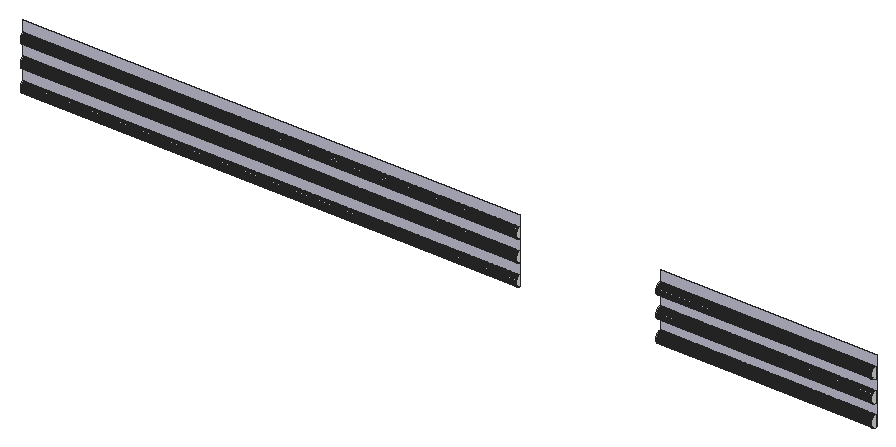
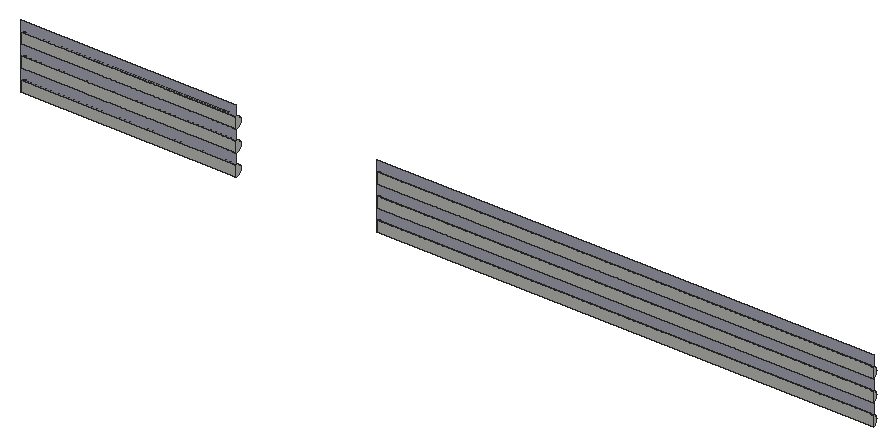
# SketchUp Ruby script. Lengths in millimetres.
U = 1.mm
M = Sketchup.active_model
def pt(a) = Geom::Point3d.new(a.map { |v| v * U })
def face(e, loops, mat)
  f = e.add_face(loops[0].map { |a| pt(a) })
  loops[1..].each { |l| e.add_face(l.map { |a| pt(a) }).erase! }
  f.material = f.back_material = mat if mat
  f
end
# faces: each face lists its corners as indices into pts; further lists are holes
def faces(e, pts, list, mat = nil) = list.each { |f| face(e, (f[0].is_a?(Array) ? f : [f]).map { |l| l.map { |i| pts[i] } }, mat) }
# xy, xz, yz: faces in a plane at the given z, y or x. An outline is a flat list of corners, or four numbers for a rectangle; further outlines are holes
def ring(l) = l.size == 4 ? [[l[0], l[1]], [l[2], l[1]], [l[2], l[3]], [l[0], l[3]]] : l.each_slice(2).to_a
def flat(e, list, mat, &to3) = list.each { |f| face(e, (f[0].is_a?(Array) ? f : [f]).map { |l| ring(l).map { |u, v| to3.(u, v) } }, mat) }
def xy(e, z, list, mat = nil) = flat(e, list, mat) { |x, y| [x, y, z] }
def xz(e, y, list, mat = nil) = flat(e, list, mat) { |x, z| [x, y, z] }
def yz(e, x, list, mat = nil) = flat(e, list, mat) { |y, z| [x, y, z] }
def lines(e, pts, list) = list.each { |a, b| e.add_line(pt(pts[a]), pt(pts[b])) }
# prism: a flat outline (further loops are holes) pulled along v
def prism(e, loops, v, mat = nil)
  f = face(e, loops, mat); d = Geom::Vector3d.new(v.map { |x| x * U })
  f.pushpull(f.normal.samedirection?(d) ? d.length : -d.length)
end
def box(e, o, s, mat = nil) = prism(e, [[o, [o[0] + s[0], o[1], o[2]], [o[0] + s[0], o[1] + s[1], o[2]], [o[0], o[1] + s[1], o[2]]]], [0, 0, s[2]], mat)
def at(x, y, z, deg = 0) = Geom::Transformation.translation(pt([x, y, z])) * Geom::Transformation.rotation(ORIGIN, Z_AXIS, deg.degrees)
def axes(o, x, y, z) = Geom::Transformation.new([*x, 0, *y, 0, *z, 0, *pt(o).to_a, 1])
def part(name) = M.definitions.add(name)
# library, detail: a bought-in or finely detailed component or shape, given as its bounding box
def library(name, o, s) = part(name).tap { |d| box(d.entities, o, s) }
def detail(e, o, s) = box(e.add_group.entities, o, s)
def put(e, d, t, mat = nil) = e.add_instance(d, t).tap { |i| i.material = mat if mat }
def group(e, t, mat = nil) = e.add_group.tap { |g| g.transformation = t; g.material = mat if mat }.entities
root = M.entities
M.materials.add("[0116_Lavender]").color = [197, 197, 214]
xz(root,16548.1,[[11038.5,6873.9,25059.3,7178.7],[29021.7,6873.9,35117.7,7178.7],[11038.5,7483.5,25059.3,7788.3],[29021.7,7483.5,35117.7,7788.3],[11038.5,8093.1,25059.3,8397.9],
  [29021.7,8093.1,35117.7,8397.9]])
xz(root,16548.1,[[11038.5,7178.7,25059.3,7483.5],[29021.7,7178.7,35117.7,7483.5],[11038.5,7788.3,25059.3,8093.1],[29021.7,7788.3,35117.7,8093.1],[11038.5,8397.9,25059.3,8702.7],
  [29021.7,8397.9,35117.7,8702.7]],"[0116_Lavender]")
yz(root,11038.5,[[16548.1,6873.9,16536.2,6879.2,16524.8,6885.5,16514,6892.6,16503.7,6900.6,16494.1,6909.4,16485.2,6918.9,16477.1,6929,16469.8,6939.8,16463.4,6951.1,16458,6962.9,16453.4,6975.1,16449.9,6987.6,16447.3,7000.4,16445.8,7013.3,16445.3,7026.3,16445.8,7039.3,16447.3,7052.2,16449.9,7064.9,16453.4,7077.4,16458,7089.6,16463.4,7101.4,16469.8,7112.7,16477.1,7123.5,16485.2,7133.7,16494.1,7143.2,16503.7,7152,16514,7159.9,16524.8,7167.1,16536.2,7173.3,16548.1,7178.7],[16548.1,7483.5,16536.2,7488.8,16524.8,7495.1,16514,7502.2,16503.7,7510.2,16494.1,7519,16485.2,7528.5,16477.1,7538.6,16469.8,7549.4,16463.4,7560.7,16458,7572.5,16453.4,7584.7,16449.9,7597.2,16447.3,7610,16445.8,7622.9,16445.3,7635.9,16445.8,7648.9,16447.3,7661.8,16449.9,7674.5,16453.4,7687,16458,7699.2,16463.4,7711,16469.8,7722.3,16477.1,7733.1,16485.2,7743.3,16494.1,7752.8,16503.7,7761.6,16514,7769.5,16524.8,7776.7,16536.2,7782.9,16548.1,7788.3],[16548.1,8093.1,16536.2,8098.4,16524.8,8104.7,16514,8111.8,16503.7,8119.8,16494.1,8128.6,16485.2,8138.1,16477.1,8148.2,16469.8,8159,16463.4,8170.3,16458,8182.1,16453.4,8194.3,16449.9,8206.8,16447.3,8219.6,16445.8,8232.5,16445.3,8245.5,16445.8,8258.5,16447.3,8271.4,16449.9,8284.1,16453.4,8296.6,16458,8308.8,16463.4,8320.6,16469.8,8331.9,16477.1,8342.7,16485.2,8352.9,16494.1,8362.4,16503.7,8371.2,16514,8379.1,16524.8,8386.3,16536.2,8392.5,16548.1,8397.9]])
yz(root,25059.3,[[16548.1,6873.9,16548.1,7178.7,16536.2,7173.3,16524.8,7167.1,16514,7159.9,16503.7,7152,16494.1,7143.2,16485.2,7133.7,16477.1,7123.5,16469.8,7112.7,16463.4,7101.4,16458,7089.6,16453.4,7077.4,16449.9,7064.9,16447.3,7052.2,16445.8,7039.3,16445.3,7026.3,16445.8,7013.3,16447.3,7000.4,16449.9,6987.6,16453.4,6975.1,16458,6962.9,16463.4,6951.1,16469.8,6939.8,16477.1,6929,16485.2,6918.9,16494.1,6909.4,16503.7,6900.6,16514,6892.6,16524.8,6885.5,16536.2,6879.2],[16548.1,7483.5,16548.1,7788.3,16536.2,7782.9,16524.8,7776.7,16514,7769.5,16503.7,7761.6,16494.1,7752.8,16485.2,7743.3,16477.1,7733.1,16469.8,7722.3,16463.4,7711,16458,7699.2,16453.4,7687,16449.9,7674.5,16447.3,7661.8,16445.8,7648.9,16445.3,7635.9,16445.8,7622.9,16447.3,7610,16449.9,7597.2,16453.4,7584.7,16458,7572.5,16463.4,7560.7,16469.8,7549.4,16477.1,7538.6,16485.2,7528.5,16494.1,7519,16503.7,7510.2,16514,7502.2,16524.8,7495.1,16536.2,7488.8],[16548.1,8093.1,16548.1,8397.9,16536.2,8392.5,16524.8,8386.3,16514,8379.1,16503.7,8371.2,16494.1,8362.4,16485.2,8352.9,16477.1,8342.7,16469.8,8331.9,16463.4,8320.6,16458,8308.8,16453.4,8296.6,16449.9,8284.1,16447.3,8271.4,16445.8,8258.5,16445.3,8245.5,16445.8,8232.5,16447.3,8219.6,16449.9,8206.8,16453.4,8194.3,16458,8182.1,16463.4,8170.3,16469.8,8159,16477.1,8148.2,16485.2,8138.1,16494.1,8128.6,16503.7,8119.8,16514,8111.8,16524.8,8104.7,16536.2,8098.4]])
yz(root,29021.7,[[16548.1,6873.9,16540.1,6874.1,16532.2,6874.7,16524.3,6875.8,16516.4,6877.2,16508.7,6879.1,16501,6881.3,16493.5,6884,16486.1,6887.1,16478.9,6890.5,16471.9,6894.3,16465.1,6898.5,16458.5,6903,16452.2,6907.8,16446.1,6913,16440.3,6918.5,16434.8,6924.3,16429.7,6930.4,16424.8,6936.7,16420.3,6943.3,16416.1,6950.1,16412.3,6957.1,16408.9,6964.3,16405.8,6971.7,16403.2,6979.2,16400.9,6986.8,16399,6994.6,16397.6,7002.4,16396.5,7010.3,16395.9,7018.3,16395.7,7026.3,16395.9,7034.3,16396.5,7042.2,16397.6,7050.1,16399,7058,16400.9,7065.7,16403.2,7073.4,16405.8,7080.9,16408.9,7088.3,16412.3,7095.5,16416.1,7102.5,16420.3,7109.3,16424.8,7115.9,16429.7,7122.2,16434.8,7128.3,16440.3,7134,16446.1,7139.5,16452.2,7144.7,16458.5,7149.6,16465.1,7154.1,16471.9,7158.3,16478.9,7162.1,16486.1,7165.5,16493.5,7168.6,16501,7171.2,16508.7,7173.5,16516.4,7175.3,16524.3,7176.8,16532.2,7177.8,16540.1,7178.5,16548.1,7178.7],[16548.1,7483.5,16540.1,7483.7,16532.2,7484.3,16524.3,7485.4,16516.4,7486.8,16508.7,7488.7,16501,7490.9,16493.5,7493.6,16486.1,7496.7,16478.9,7500.1,16471.9,7503.9,16465.1,7508.1,16458.5,7512.6,16452.2,7517.4,16446.1,7522.6,16440.3,7528.1,16434.8,7533.9,16429.7,7540,16424.8,7546.3,16420.3,7552.9,16416.1,7559.7,16412.3,7566.7,16408.9,7573.9,16405.8,7581.3,16403.2,7588.8,16400.9,7596.4,16399,7604.2,16397.6,7612,16396.5,7619.9,16395.9,7627.9,16395.7,7635.9,16395.9,7643.9,16396.5,7651.8,16397.6,7659.7,16399,7667.6,16400.9,7675.3,16403.2,7683,16405.8,7690.5,16408.9,7697.9,16412.3,7705.1,16416.1,7712.1,16420.3,7718.9,16424.8,7725.5,16429.7,7731.8,16434.8,7737.9,16440.3,7743.6,16446.1,7749.1,16452.2,7754.3,16458.5,7759.2,16465.1,7763.7,16471.9,7767.9,16478.9,7771.7,16486.1,7775.1,16493.5,7778.2,16501,7780.8,16508.7,7783.1,16516.4,7784.9,16524.3,7786.4,16532.2,7787.4,16540.1,7788.1,16548.1,7788.3],[16548.1,8093.1,16540.1,8093.3,16532.2,8093.9,16524.3,8095,16516.4,8096.4,16508.7,8098.3,16501,8100.5,16493.5,8103.2,16486.1,8106.3,16478.9,8109.7,16471.9,8113.5,16465.1,8117.7,16458.5,8122.2,16452.2,8127,16446.1,8132.2,16440.3,8137.7,16434.8,8143.5,16429.7,8149.6,16424.8,8155.9,16420.3,8162.5,16416.1,8169.3,16412.3,8176.3,16408.9,8183.5,16405.8,8190.9,16403.2,8198.4,16400.9,8206,16399,8213.8,16397.6,8221.6,16396.5,8229.5,16395.9,8237.5,16395.7,8245.5,16395.9,8253.5,16396.5,8261.4,16397.6,8269.3,16399,8277.2,16400.9,8284.9,16403.2,8292.6,16405.8,8300.1,16408.9,8307.5,16412.3,8314.7,16416.1,8321.7,16420.3,8328.5,16424.8,8335.1,16429.7,8341.4,16434.8,8347.5,16440.3,8353.2,16446.1,8358.7,16452.2,8363.9,16458.5,8368.8,16465.1,8373.3,16471.9,8377.5,16478.9,8381.3,16486.1,8384.7,16493.5,8387.8,16501,8390.4,16508.7,8392.7,16516.4,8394.5,16524.3,8396,16532.2,8397,16540.1,8397.7,16548.1,8397.9]])
yz(root,35117.7,[[16548.1,6873.9,16548.1,7178.7,16540.1,7178.5,16532.2,7177.8,16524.3,7176.8,16516.4,7175.3,16508.7,7173.5,16501,7171.2,16493.5,7168.6,16486.1,7165.5,16478.9,7162.1,16471.9,7158.3,16465.1,7154.1,16458.5,7149.6,16452.2,7144.7,16446.1,7139.5,16440.3,7134,16434.8,7128.3,16429.7,7122.2,16424.8,7115.9,16420.3,7109.3,16416.1,7102.5,16412.3,7095.5,16408.9,7088.3,16405.8,7080.9,16403.2,7073.4,16400.9,7065.7,16399,7058,16397.6,7050.1,16396.5,7042.2,16395.9,7034.3,16395.7,7026.3,16395.9,7018.3,16396.5,7010.3,16397.6,7002.4,16399,6994.6,16400.9,6986.8,16403.2,6979.2,16405.8,6971.7,16408.9,6964.3,16412.3,6957.1,16416.1,6950.1,16420.3,6943.3,16424.8,6936.7,16429.7,6930.4,16434.8,6924.3,16440.3,6918.5,16446.1,6913,16452.2,6907.8,16458.5,6903,16465.1,6898.5,16471.9,6894.3,16478.9,6890.5,16486.1,6887.1,16493.5,6884,16501,6881.3,16508.7,6879.1,16516.4,6877.2,16524.3,6875.8,16532.2,6874.7,16540.1,6874.1],[16548.1,7483.5,16548.1,7788.3,16540.1,7788.1,16532.2,7787.4,16524.3,7786.4,16516.4,7784.9,16508.7,7783.1,16501,7780.8,16493.5,7778.2,16486.1,7775.1,16478.9,7771.7,16471.9,7767.9,16465.1,7763.7,16458.5,7759.2,16452.2,7754.3,16446.1,7749.1,16440.3,7743.6,16434.8,7737.9,16429.7,7731.8,16424.8,7725.5,16420.3,7718.9,16416.1,7712.1,16412.3,7705.1,16408.9,7697.9,16405.8,7690.5,16403.2,7683,16400.9,7675.3,16399,7667.6,16397.6,7659.7,16396.5,7651.8,16395.9,7643.9,16395.7,7635.9,16395.9,7627.9,16396.5,7619.9,16397.6,7612,16399,7604.2,16400.9,7596.4,16403.2,7588.8,16405.8,7581.3,16408.9,7573.9,16412.3,7566.7,16416.1,7559.7,16420.3,7552.9,16424.8,7546.3,16429.7,7540,16434.8,7533.9,16440.3,7528.1,16446.1,7522.6,16452.2,7517.4,16458.5,7512.6,16465.1,7508.1,16471.9,7503.9,16478.9,7500.1,16486.1,7496.7,16493.5,7493.6,16501,7490.9,16508.7,7488.7,16516.4,7486.8,16524.3,7485.4,16532.2,7484.3,16540.1,7483.7],[16548.1,8093.1,16548.1,8397.9,16540.1,8397.7,16532.2,8397,16524.3,8396,16516.4,8394.5,16508.7,8392.7,16501,8390.4,16493.5,8387.8,16486.1,8384.7,16478.9,8381.3,16471.9,8377.5,16465.1,8373.3,16458.5,8368.8,16452.2,8363.9,16446.1,8358.7,16440.3,8353.2,16434.8,8347.5,16429.7,8341.4,16424.8,8335.1,16420.3,8328.5,16416.1,8321.7,16412.3,8314.7,16408.9,8307.5,16405.8,8300.1,16403.2,8292.6,16400.9,8284.9,16399,8277.2,16397.6,8269.3,16396.5,8261.4,16395.9,8253.5,16395.7,8245.5,16395.9,8237.5,16396.5,8229.5,16397.6,8221.6,16399,8213.8,16400.9,8206,16403.2,8198.4,16405.8,8190.9,16408.9,8183.5,16412.3,8176.3,16416.1,8169.3,16420.3,8162.5,16424.8,8155.9,16429.7,8149.6,16434.8,8143.5,16440.3,8137.7,16446.1,8132.2,16452.2,8127,16458.5,8122.2,16465.1,8117.7,16471.9,8113.5,16478.9,8109.7,16486.1,8106.3,16493.5,8103.2,16501,8100.5,16508.7,8098.3,16516.4,8096.4,16524.3,8095,16532.2,8093.9,16540.1,8093.3]])
p = [[25059.3,16548.1,6873.9],[25059.3,16536.2,6879.2],[11038.5,16536.2,6879.2],[11038.5,16548.1,6873.9],[35117.7,16548.1,6873.9],[35117.7,16540.1,6874.1],
  [29021.7,16540.1,6874.1],[29021.7,16548.1,6873.9],[35117.7,16532.2,6874.7],[29021.7,16532.2,6874.7],[35117.7,16524.3,6875.8],[29021.7,16524.3,6875.8],
  [35117.7,16516.4,6877.2],[29021.7,16516.4,6877.2],[35117.7,16508.7,6879.1],[29021.7,16508.7,6879.1],[35117.7,16501,6881.3],[29021.7,16501,6881.3],
  [25059.3,16524.8,6885.5],[11038.5,16524.8,6885.5],[35117.7,16493.5,6884],[29021.7,16493.5,6884],[35117.7,16486.1,6887.1],[29021.7,16486.1,6887.1],
  [25059.3,16514,6892.6],[11038.5,16514,6892.6],[35117.7,16478.9,6890.5],[29021.7,16478.9,6890.5],[35117.7,16471.9,6894.3],[29021.7,16471.9,6894.3],
  [25059.3,16503.7,6900.6],[11038.5,16503.7,6900.6],[35117.7,16465.1,6898.5],[29021.7,16465.1,6898.5],[35117.7,16458.5,6903],[29021.7,16458.5,6903],
  [25059.3,16494.1,6909.4],[11038.5,16494.1,6909.4],[35117.7,16452.2,6907.8],[29021.7,16452.2,6907.8],[35117.7,16446.1,6913],[29021.7,16446.1,6913],
  [25059.3,16485.2,6918.9],[11038.5,16485.2,6918.9],[35117.7,16440.3,6918.5],[29021.7,16440.3,6918.5],[35117.7,16434.8,6924.3],[29021.7,16434.8,6924.3],
  [25059.3,16477.1,6929],[11038.5,16477.1,6929],[35117.7,16429.7,6930.4],[29021.7,16429.7,6930.4],[25059.3,16469.8,6939.8],[11038.5,16469.8,6939.8],
  [35117.7,16424.8,6936.7],[29021.7,16424.8,6936.7],[35117.7,16420.3,6943.3],[29021.7,16420.3,6943.3],[25059.3,16463.4,6951.1],[11038.5,16463.4,6951.1],
  [35117.7,16416.1,6950.1],[29021.7,16416.1,6950.1],[35117.7,16412.3,6957.1],[29021.7,16412.3,6957.1],[25059.3,16458,6962.9],[11038.5,16458,6962.9],
  [35117.7,16408.9,6964.3],[29021.7,16408.9,6964.3],[25059.3,16453.4,6975.1],[11038.5,16453.4,6975.1],[35117.7,16405.8,6971.7],[29021.7,16405.8,6971.7],
  [35117.7,16403.2,6979.2],[29021.7,16403.2,6979.2],[25059.3,16449.9,6987.6],[11038.5,16449.9,6987.6],[35117.7,16400.9,6986.8],[29021.7,16400.9,6986.8],
  [35117.7,16399,6994.6],[29021.7,16399,6994.6],[25059.3,16447.3,7000.4],[11038.5,16447.3,7000.4],[35117.7,16397.6,7002.4],[29021.7,16397.6,7002.4],
  [25059.3,16445.8,7013.3],[11038.5,16445.8,7013.3],[35117.7,16396.5,7010.3],[29021.7,16396.5,7010.3],[35117.7,16395.9,7018.3],[29021.7,16395.9,7018.3],
  [25059.3,16445.3,7026.3],[11038.5,16445.3,7026.3],[35117.7,16395.7,7026.3],[29021.7,16395.7,7026.3],[35117.7,16395.9,7034.3],[29021.7,16395.9,7034.3],
  [25059.3,16445.8,7039.3],[11038.5,16445.8,7039.3],[35117.7,16396.5,7042.2],[29021.7,16396.5,7042.2],[25059.3,16447.3,7052.2],[11038.5,16447.3,7052.2],
  [35117.7,16397.6,7050.1],[29021.7,16397.6,7050.1],[35117.7,16399,7058],[29021.7,16399,7058],[25059.3,16449.9,7064.9],[11038.5,16449.9,7064.9],
  [35117.7,16400.9,7065.7],[29021.7,16400.9,7065.7],[25059.3,16453.4,7077.4],[11038.5,16453.4,7077.4],[35117.7,16403.2,7073.4],[29021.7,16403.2,7073.4],
  [35117.7,16405.8,7080.9],[29021.7,16405.8,7080.9],[25059.3,16458,7089.6],[11038.5,16458,7089.6],[35117.7,16408.9,7088.3],[29021.7,16408.9,7088.3],
  [35117.7,16412.3,7095.5],[29021.7,16412.3,7095.5],[25059.3,16463.4,7101.4],[11038.5,16463.4,7101.4],[35117.7,16416.1,7102.5],[29021.7,16416.1,7102.5],
  [25059.3,16469.8,7112.7],[11038.5,16469.8,7112.7],[35117.7,16420.3,7109.3],[29021.7,16420.3,7109.3],[35117.7,16424.8,7115.9],[29021.7,16424.8,7115.9],
  [25059.3,16477.1,7123.5],[11038.5,16477.1,7123.5],[35117.7,16429.7,7122.2],[29021.7,16429.7,7122.2],[35117.7,16434.8,7128.3],[29021.7,16434.8,7128.3],
  [25059.3,16485.2,7133.7],[11038.5,16485.2,7133.7],[35117.7,16440.3,7134],[29021.7,16440.3,7134],[25059.3,16494.1,7143.2],[11038.5,16494.1,7143.2],
  [35117.7,16446.1,7139.5],[29021.7,16446.1,7139.5],[35117.7,16452.2,7144.7],[29021.7,16452.2,7144.7],[25059.3,16503.7,7152],[11038.5,16503.7,7152],
  [35117.7,16458.5,7149.6],[29021.7,16458.5,7149.6],[35117.7,16465.1,7154.1],[29021.7,16465.1,7154.1],[25059.3,16514,7159.9],[11038.5,16514,7159.9],
  [35117.7,16471.9,7158.3],[29021.7,16471.9,7158.3],[35117.7,16478.9,7162.1],[29021.7,16478.9,7162.1],[25059.3,16524.8,7167.1],[11038.5,16524.8,7167.1],
  [35117.7,16486.1,7165.5],[29021.7,16486.1,7165.5],[35117.7,16493.5,7168.6],[29021.7,16493.5,7168.6],[25059.3,16536.2,7173.3],[11038.5,16536.2,7173.3],
  [35117.7,16501,7171.2],[29021.7,16501,7171.2],[35117.7,16508.7,7173.5],[29021.7,16508.7,7173.5],[25059.3,16548.1,7178.7],[11038.5,16548.1,7178.7],
  [35117.7,16516.4,7175.3],[29021.7,16516.4,7175.3],[35117.7,16524.3,7176.8],[29021.7,16524.3,7176.8],[35117.7,16532.2,7177.8],[29021.7,16532.2,7177.8],
  [35117.7,16540.1,7178.5],[29021.7,16540.1,7178.5],[35117.7,16548.1,7178.7],[29021.7,16548.1,7178.7],[25059.3,16548.1,7483.5],[25059.3,16536.2,7488.8],
  [11038.5,16536.2,7488.8],[11038.5,16548.1,7483.5],[35117.7,16548.1,7483.5],[35117.7,16540.1,7483.7],[29021.7,16540.1,7483.7],[29021.7,16548.1,7483.5],
  [35117.7,16532.2,7484.3],[29021.7,16532.2,7484.3],[35117.7,16524.3,7485.4],[29021.7,16524.3,7485.4],[35117.7,16516.4,7486.8],[29021.7,16516.4,7486.8],
  [35117.7,16508.7,7488.7],[29021.7,16508.7,7488.7],[35117.7,16501,7490.9],[29021.7,16501,7490.9],[25059.3,16524.8,7495.1],[11038.5,16524.8,7495.1],
  [35117.7,16493.5,7493.6],[29021.7,16493.5,7493.6],[35117.7,16486.1,7496.7],[29021.7,16486.1,7496.7],[25059.3,16514,7502.2],[11038.5,16514,7502.2],
  [35117.7,16478.9,7500.1],[29021.7,16478.9,7500.1],[35117.7,16471.9,7503.9],[29021.7,16471.9,7503.9],[25059.3,16503.7,7510.2],[11038.5,16503.7,7510.2],
  [35117.7,16465.1,7508.1],[29021.7,16465.1,7508.1],[35117.7,16458.5,7512.6],[29021.7,16458.5,7512.6],[25059.3,16494.1,7519],[11038.5,16494.1,7519],
  [35117.7,16452.2,7517.4],[29021.7,16452.2,7517.4],[35117.7,16446.1,7522.6],[29021.7,16446.1,7522.6],[25059.3,16485.2,7528.5],[11038.5,16485.2,7528.5],
  [35117.7,16440.3,7528.1],[29021.7,16440.3,7528.1],[35117.7,16434.8,7533.9],[29021.7,16434.8,7533.9],[25059.3,16477.1,7538.6],[11038.5,16477.1,7538.6],
  [35117.7,16429.7,7540],[29021.7,16429.7,7540],[25059.3,16469.8,7549.4],[11038.5,16469.8,7549.4],[35117.7,16424.8,7546.3],[29021.7,16424.8,7546.3],
  [35117.7,16420.3,7552.9],[29021.7,16420.3,7552.9],[25059.3,16463.4,7560.7],[11038.5,16463.4,7560.7],[35117.7,16416.1,7559.7],[29021.7,16416.1,7559.7],
  [35117.7,16412.3,7566.7],[29021.7,16412.3,7566.7],[25059.3,16458,7572.5],[11038.5,16458,7572.5],[35117.7,16408.9,7573.9],[29021.7,16408.9,7573.9],
  [25059.3,16453.4,7584.7],[11038.5,16453.4,7584.7],[35117.7,16405.8,7581.3],[29021.7,16405.8,7581.3],[35117.7,16403.2,7588.8],[29021.7,16403.2,7588.8],
  [25059.3,16449.9,7597.2],[11038.5,16449.9,7597.2],[35117.7,16400.9,7596.4],[29021.7,16400.9,7596.4],[35117.7,16399,7604.2],[29021.7,16399,7604.2],
  [25059.3,16447.3,7610],[11038.5,16447.3,7610],[35117.7,16397.6,7612],[29021.7,16397.6,7612],[25059.3,16445.8,7622.9],[11038.5,16445.8,7622.9],
  [35117.7,16396.5,7619.9],[29021.7,16396.5,7619.9],[35117.7,16395.9,7627.9],[29021.7,16395.9,7627.9],[25059.3,16445.3,7635.9],[11038.5,16445.3,7635.9],
  [35117.7,16395.7,7635.9],[29021.7,16395.7,7635.9],[35117.7,16395.9,7643.9],[29021.7,16395.9,7643.9],[25059.3,16445.8,7648.9],[11038.5,16445.8,7648.9],
  [35117.7,16396.5,7651.8],[29021.7,16396.5,7651.8],[25059.3,16447.3,7661.8],[11038.5,16447.3,7661.8],[35117.7,16397.6,7659.7],[29021.7,16397.6,7659.7],
  [35117.7,16399,7667.6],[29021.7,16399,7667.6],[25059.3,16449.9,7674.5],[11038.5,16449.9,7674.5],[35117.7,16400.9,7675.3],[29021.7,16400.9,7675.3],
  [25059.3,16453.4,7687],[11038.5,16453.4,7687],[35117.7,16403.2,7683],[29021.7,16403.2,7683],[35117.7,16405.8,7690.5],[29021.7,16405.8,7690.5],
  [25059.3,16458,7699.2],[11038.5,16458,7699.2],[35117.7,16408.9,7697.9],[29021.7,16408.9,7697.9],[35117.7,16412.3,7705.1],[29021.7,16412.3,7705.1],
  [25059.3,16463.4,7711],[11038.5,16463.4,7711],[35117.7,16416.1,7712.1],[29021.7,16416.1,7712.1],[25059.3,16469.8,7722.3],[11038.5,16469.8,7722.3],
  [35117.7,16420.3,7718.9],[29021.7,16420.3,7718.9],[35117.7,16424.8,7725.5],[29021.7,16424.8,7725.5],[25059.3,16477.1,7733.1],[11038.5,16477.1,7733.1],
  [35117.7,16429.7,7731.8],[29021.7,16429.7,7731.8],[35117.7,16434.8,7737.9],[29021.7,16434.8,7737.9],[25059.3,16485.2,7743.3],[11038.5,16485.2,7743.3],
  [35117.7,16440.3,7743.6],[29021.7,16440.3,7743.6],[25059.3,16494.1,7752.8],[11038.5,16494.1,7752.8],[35117.7,16446.1,7749.1],[29021.7,16446.1,7749.1],
  [35117.7,16452.2,7754.3],[29021.7,16452.2,7754.3],[25059.3,16503.7,7761.6],[11038.5,16503.7,7761.6],[35117.7,16458.5,7759.2],[29021.7,16458.5,7759.2],
  [35117.7,16465.1,7763.7],[29021.7,16465.1,7763.7],[25059.3,16514,7769.5],[11038.5,16514,7769.5],[35117.7,16471.9,7767.9],[29021.7,16471.9,7767.9],
  [35117.7,16478.9,7771.7],[29021.7,16478.9,7771.7],[25059.3,16524.8,7776.7],[11038.5,16524.8,7776.7],[35117.7,16486.1,7775.1],[29021.7,16486.1,7775.1],
  [35117.7,16493.5,7778.2],[29021.7,16493.5,7778.2],[25059.3,16536.2,7782.9],[11038.5,16536.2,7782.9],[35117.7,16501,7780.8],[29021.7,16501,7780.8],
  [35117.7,16508.7,7783.1],[29021.7,16508.7,7783.1],[25059.3,16548.1,7788.3],[11038.5,16548.1,7788.3],[35117.7,16516.4,7784.9],[29021.7,16516.4,7784.9],
  [35117.7,16524.3,7786.4],[29021.7,16524.3,7786.4],[35117.7,16532.2,7787.4],[29021.7,16532.2,7787.4],[35117.7,16540.1,7788.1],[29021.7,16540.1,7788.1],
  [35117.7,16548.1,7788.3],[29021.7,16548.1,7788.3],[25059.3,16548.1,8093.1],[25059.3,16536.2,8098.4],[11038.5,16536.2,8098.4],[11038.5,16548.1,8093.1],
  [35117.7,16548.1,8093.1],[35117.7,16540.1,8093.3],[29021.7,16540.1,8093.3],[29021.7,16548.1,8093.1],[35117.7,16532.2,8093.9],[29021.7,16532.2,8093.9],
  [35117.7,16524.3,8095],[29021.7,16524.3,8095],[35117.7,16516.4,8096.4],[29021.7,16516.4,8096.4],[35117.7,16508.7,8098.3],[29021.7,16508.7,8098.3],
  [35117.7,16501,8100.5],[29021.7,16501,8100.5],[25059.3,16524.8,8104.7],[11038.5,16524.8,8104.7],[35117.7,16493.5,8103.2],[29021.7,16493.5,8103.2],
  [35117.7,16486.1,8106.3],[29021.7,16486.1,8106.3],[25059.3,16514,8111.8],[11038.5,16514,8111.8],[35117.7,16478.9,8109.7],[29021.7,16478.9,8109.7],
  [35117.7,16471.9,8113.5],[29021.7,16471.9,8113.5],[25059.3,16503.7,8119.8],[11038.5,16503.7,8119.8],[35117.7,16465.1,8117.7],[29021.7,16465.1,8117.7],
  [35117.7,16458.5,8122.2],[29021.7,16458.5,8122.2],[25059.3,16494.1,8128.6],[11038.5,16494.1,8128.6],[35117.7,16452.2,8127],[29021.7,16452.2,8127],
  [35117.7,16446.1,8132.2],[29021.7,16446.1,8132.2],[25059.3,16485.2,8138.1],[11038.5,16485.2,8138.1],[35117.7,16440.3,8137.7],[29021.7,16440.3,8137.7],
  [35117.7,16434.8,8143.5],[29021.7,16434.8,8143.5],[25059.3,16477.1,8148.2],[11038.5,16477.1,8148.2],[35117.7,16429.7,8149.6],[29021.7,16429.7,8149.6],
  [25059.3,16469.8,8159],[11038.5,16469.8,8159],[35117.7,16424.8,8155.9],[29021.7,16424.8,8155.9],[35117.7,16420.3,8162.5],[29021.7,16420.3,8162.5],
  [25059.3,16463.4,8170.3],[11038.5,16463.4,8170.3],[35117.7,16416.1,8169.3],[29021.7,16416.1,8169.3],[35117.7,16412.3,8176.3],[29021.7,16412.3,8176.3],
  [25059.3,16458,8182.1],[11038.5,16458,8182.1],[35117.7,16408.9,8183.5],[29021.7,16408.9,8183.5],[25059.3,16453.4,8194.3],[11038.5,16453.4,8194.3],
  [35117.7,16405.8,8190.9],[29021.7,16405.8,8190.9],[35117.7,16403.2,8198.4],[29021.7,16403.2,8198.4],[25059.3,16449.9,8206.8],[11038.5,16449.9,8206.8],
  [35117.7,16400.9,8206],[29021.7,16400.9,8206],[35117.7,16399,8213.8],[29021.7,16399,8213.8],[25059.3,16447.3,8219.6],[11038.5,16447.3,8219.6],
  [35117.7,16397.6,8221.6],[29021.7,16397.6,8221.6],[25059.3,16445.8,8232.5],[11038.5,16445.8,8232.5],[35117.7,16396.5,8229.5],[29021.7,16396.5,8229.5],
  [35117.7,16395.9,8237.5],[29021.7,16395.9,8237.5],[25059.3,16445.3,8245.5],[11038.5,16445.3,8245.5],[35117.7,16395.7,8245.5],[29021.7,16395.7,8245.5],
  [35117.7,16395.9,8253.5],[29021.7,16395.9,8253.5],[25059.3,16445.8,8258.5],[11038.5,16445.8,8258.5],[35117.7,16396.5,8261.4],[29021.7,16396.5,8261.4],
  [25059.3,16447.3,8271.4],[11038.5,16447.3,8271.4],[35117.7,16397.6,8269.3],[29021.7,16397.6,8269.3],[35117.7,16399,8277.2],[29021.7,16399,8277.2],
  [25059.3,16449.9,8284.1],[11038.5,16449.9,8284.1],[35117.7,16400.9,8284.9],[29021.7,16400.9,8284.9],[25059.3,16453.4,8296.6],[11038.5,16453.4,8296.6],
  [35117.7,16403.2,8292.6],[29021.7,16403.2,8292.6],[35117.7,16405.8,8300.1],[29021.7,16405.8,8300.1],[25059.3,16458,8308.8],[11038.5,16458,8308.8],
  [35117.7,16408.9,8307.5],[29021.7,16408.9,8307.5],[35117.7,16412.3,8314.7],[29021.7,16412.3,8314.7],[25059.3,16463.4,8320.6],[11038.5,16463.4,8320.6],
  [35117.7,16416.1,8321.7],[29021.7,16416.1,8321.7],[25059.3,16469.8,8331.9],[11038.5,16469.8,8331.9],[35117.7,16420.3,8328.5],[29021.7,16420.3,8328.5],
  [35117.7,16424.8,8335.1],[29021.7,16424.8,8335.1],[25059.3,16477.1,8342.7],[11038.5,16477.1,8342.7],[35117.7,16429.7,8341.4],[29021.7,16429.7,8341.4],
  [35117.7,16434.8,8347.5],[29021.7,16434.8,8347.5],[25059.3,16485.2,8352.9],[11038.5,16485.2,8352.9],[35117.7,16440.3,8353.2],[29021.7,16440.3,8353.2],
  [25059.3,16494.1,8362.4],[11038.5,16494.1,8362.4],[35117.7,16446.1,8358.7],[29021.7,16446.1,8358.7],[35117.7,16452.2,8363.9],[29021.7,16452.2,8363.9],
  [25059.3,16503.7,8371.2],[11038.5,16503.7,8371.2],[35117.7,16458.5,8368.8],[29021.7,16458.5,8368.8],[35117.7,16465.1,8373.3],[29021.7,16465.1,8373.3],
  [25059.3,16514,8379.1],[11038.5,16514,8379.1],[35117.7,16471.9,8377.5],[29021.7,16471.9,8377.5],[35117.7,16478.9,8381.3],[29021.7,16478.9,8381.3],
  [25059.3,16524.8,8386.3],[11038.5,16524.8,8386.3],[35117.7,16486.1,8384.7],[29021.7,16486.1,8384.7],[35117.7,16493.5,8387.8],[29021.7,16493.5,8387.8],
  [25059.3,16536.2,8392.5],[11038.5,16536.2,8392.5],[35117.7,16501,8390.4],[29021.7,16501,8390.4],[35117.7,16508.7,8392.7],[29021.7,16508.7,8392.7],
  [25059.3,16548.1,8397.9],[11038.5,16548.1,8397.9],[35117.7,16516.4,8394.5],[29021.7,16516.4,8394.5],[35117.7,16524.3,8396],[29021.7,16524.3,8396],
  [35117.7,16532.2,8397],[29021.7,16532.2,8397],[35117.7,16540.1,8397.7],[29021.7,16540.1,8397.7],[35117.7,16548.1,8397.9],[29021.7,16548.1,8397.9]]
faces(root,p,[[0,1,2,3],[4,5,6,7],[5,8,9,6],[8,10,11,9],[10,12,13,11],[12,14,15,13],[14,16,17,15],[1,18,19,2],
  [16,20,21,17],[20,22,23,21],[18,24,25,19],[22,26,27,23],[26,28,29,27],[24,30,31,25],[28,32,33,29],[32,34,35,33],
  [30,36,37,31],[34,38,39,35],[38,40,41,39],[36,42,43,37],[40,44,45,41],[44,46,47,45],[42,48,49,43],[46,50,51,47],
  [48,52,53,49],[50,54,55,51],[54,56,57,55],[52,58,59,53],[56,60,61,57],[60,62,63,61],[58,64,65,59],[62,66,67,63],
  [64,68,69,65],[66,70,71,67],[70,72,73,71],[68,74,75,69],[72,76,77,73],[76,78,79,77],[74,80,81,75],[78,82,83,79],
  [80,84,85,81],[82,86,87,83],[86,88,89,87],[84,90,91,85],[88,92,93,89],[92,94,95,93],[90,96,97,91],[94,98,99,95],
  [96,100,101,97],[98,102,103,99],[102,104,105,103],[100,106,107,101],[104,108,109,105],[106,110,111,107],[108,112,113,109],[112,114,115,113],
  [110,116,117,111],[114,118,119,115],[118,120,121,119],[116,122,123,117],[120,124,125,121],[122,126,127,123],[124,128,129,125],[128,130,131,129],
  [126,132,133,127],[130,134,135,131],[134,136,137,135],[132,138,139,133],[136,140,141,137],[138,142,143,139],[140,144,145,141],[144,146,147,145],
  [142,148,149,143],[146,150,151,147],[150,152,153,151],[148,154,155,149],[152,156,157,153],[156,158,159,157],[154,160,161,155],[158,162,163,159],
  [162,164,165,163],[160,166,167,161],[164,168,169,165],[168,170,171,169],[166,172,173,167],[170,174,175,171],[174,176,177,175],[176,178,179,177],
  [178,180,181,179],[180,182,183,181],[184,185,186,187],[188,189,190,191],[189,192,193,190],[192,194,195,193],[194,196,197,195],[196,198,199,197],
  [198,200,201,199],[185,202,203,186],[200,204,205,201],[204,206,207,205],[202,208,209,203],[206,210,211,207],[210,212,213,211],[208,214,215,209],
  [212,216,217,213],[216,218,219,217],[214,220,221,215],[218,222,223,219],[222,224,225,223],[220,226,227,221],[224,228,229,225],[228,230,231,229],
  [226,232,233,227],[230,234,235,231],[232,236,237,233],[234,238,239,235],[238,240,241,239],[236,242,243,237],[240,244,245,241],[244,246,247,245],
  [242,248,249,243],[246,250,251,247],[248,252,253,249],[250,254,255,251],[254,256,257,255],[252,258,259,253],[256,260,261,257],[260,262,263,261],
  [258,264,265,259],[262,266,267,263],[264,268,269,265],[266,270,271,267],[270,272,273,271],[268,274,275,269],[272,276,277,273],[276,278,279,277],
  [274,280,281,275],[278,282,283,279],[280,284,285,281],[282,286,287,283],[286,288,289,287],[284,290,291,285],[288,292,293,289],[290,294,295,291],
  [292,296,297,293],[296,298,299,297],[294,300,301,295],[298,302,303,299],[302,304,305,303],[300,306,307,301],[304,308,309,305],[306,310,311,307],
  [308,312,313,309],[312,314,315,313],[310,316,317,311],[314,318,319,315],[318,320,321,319],[316,322,323,317],[320,324,325,321],[322,326,327,323],
  [324,328,329,325],[328,330,331,329],[326,332,333,327],[330,334,335,331],[334,336,337,335],[332,338,339,333],[336,340,341,337],[340,342,343,341],
  [338,344,345,339],[342,346,347,343],[346,348,349,347],[344,350,351,345],[348,352,353,349],[352,354,355,353],[350,356,357,351],[354,358,359,355],
  [358,360,361,359],[360,362,363,361],[362,364,365,363],[364,366,367,365],[368,369,370,371],[372,373,374,375],[373,376,377,374],[376,378,379,377],
  [378,380,381,379],[380,382,383,381],[382,384,385,383],[369,386,387,370],[384,388,389,385],[388,390,391,389],[386,392,393,387],[390,394,395,391],
  [394,396,397,395],[392,398,399,393],[396,400,401,397],[400,402,403,401],[398,404,405,399],[402,406,407,403],[406,408,409,407],[404,410,411,405],
  [408,412,413,409],[412,414,415,413],[410,416,417,411],[414,418,419,415],[416,420,421,417],[418,422,423,419],[422,424,425,423],[420,426,427,421],
  [424,428,429,425],[428,430,431,429],[426,432,433,427],[430,434,435,431],[432,436,437,433],[434,438,439,435],[438,440,441,439],[436,442,443,437],
  [440,444,445,441],[444,446,447,445],[442,448,449,443],[446,450,451,447],[448,452,453,449],[450,454,455,451],[454,456,457,455],[452,458,459,453],
  [456,460,461,457],[460,462,463,461],[458,464,465,459],[462,466,467,463],[464,468,469,465],[466,470,471,467],[470,472,473,471],[468,474,475,469],
  [472,476,477,473],[474,478,479,475],[476,480,481,477],[480,482,483,481],[478,484,485,479],[482,486,487,483],[486,488,489,487],[484,490,491,485],
  [488,492,493,489],[490,494,495,491],[492,496,497,493],[496,498,499,497],[494,500,501,495],[498,502,503,499],[502,504,505,503],[500,506,507,501],
  [504,508,509,505],[506,510,511,507],[508,512,513,509],[512,514,515,513],[510,516,517,511],[514,518,519,515],[518,520,521,519],[516,522,523,517],
  [520,524,525,521],[524,526,527,525],[522,528,529,523],[526,530,531,527],[530,532,533,531],[528,534,535,529],[532,536,537,533],[536,538,539,537],
  [534,540,541,535],[538,542,543,539],[542,544,545,543],[544,546,547,545],[546,548,549,547],[548,550,551,549]],"[0116_Lavender]")
